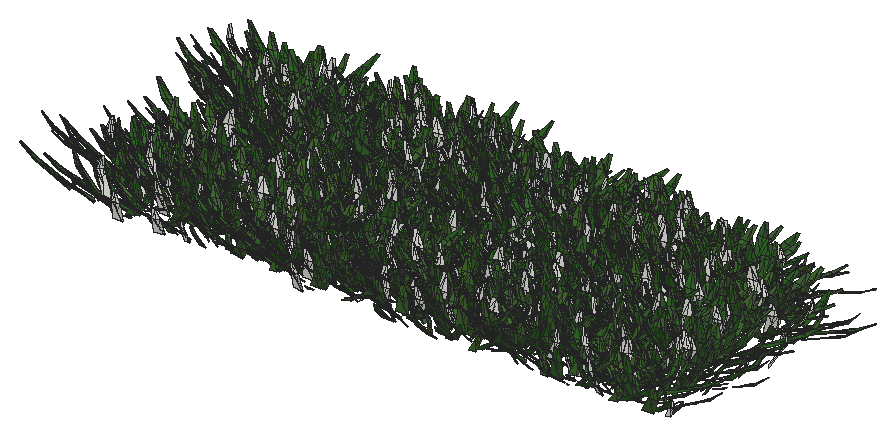
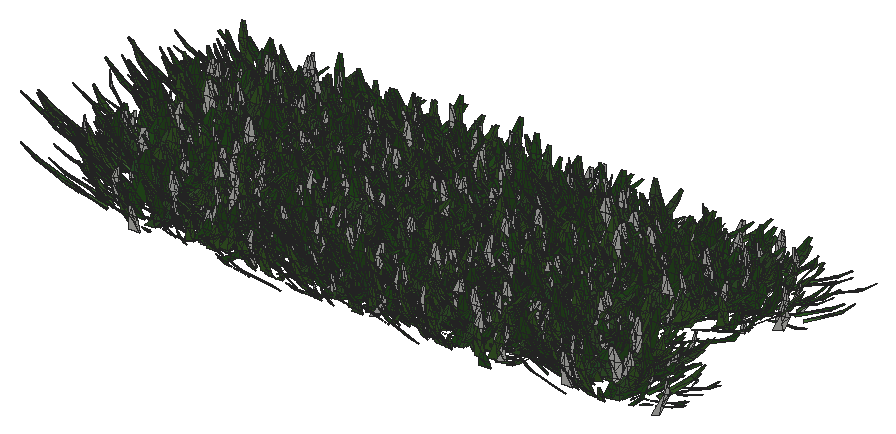
# SketchUp Ruby script. Lengths in inches.
U = 1.inch
M = Sketchup.active_model
def pt(a) = Geom::Point3d.new(a.map { |v| v * U })
def face(e, loops, mat)
  f = e.add_face(loops[0].map { |a| pt(a) })
  loops[1..].each { |l| e.add_face(l.map { |a| pt(a) }).erase! }
  f.material = f.back_material = mat if mat
  f
end
# faces: each face lists its corners as indices into pts; further lists are holes
def faces(e, pts, list, mat = nil) = list.each { |f| face(e, (f[0].is_a?(Array) ? f : [f]).map { |l| l.map { |i| pts[i] } }, mat) }
# xy, xz, yz: faces in a plane at the given z, y or x. An outline is a flat list of corners, or four numbers for a rectangle; further outlines are holes
def ring(l) = l.size == 4 ? [[l[0], l[1]], [l[2], l[1]], [l[2], l[3]], [l[0], l[3]]] : l.each_slice(2).to_a
def flat(e, list, mat, &to3) = list.each { |f| face(e, (f[0].is_a?(Array) ? f : [f]).map { |l| ring(l).map { |u, v| to3.(u, v) } }, mat) }
def xy(e, z, list, mat = nil) = flat(e, list, mat) { |x, y| [x, y, z] }
def xz(e, y, list, mat = nil) = flat(e, list, mat) { |x, z| [x, y, z] }
def yz(e, x, list, mat = nil) = flat(e, list, mat) { |y, z| [x, y, z] }
def lines(e, pts, list) = list.each { |a, b| e.add_line(pt(pts[a]), pt(pts[b])) }
# prism: a flat outline (further loops are holes) pulled along v
def prism(e, loops, v, mat = nil)
  f = face(e, loops, mat); d = Geom::Vector3d.new(v.map { |x| x * U })
  f.pushpull(f.normal.samedirection?(d) ? d.length : -d.length)
end
def box(e, o, s, mat = nil) = prism(e, [[o, [o[0] + s[0], o[1], o[2]], [o[0] + s[0], o[1] + s[1], o[2]], [o[0], o[1] + s[1], o[2]]]], [0, 0, s[2]], mat)
def at(x, y, z, deg = 0) = Geom::Transformation.translation(pt([x, y, z])) * Geom::Transformation.rotation(ORIGIN, Z_AXIS, deg.degrees)
def axes(o, x, y, z) = Geom::Transformation.new([*x, 0, *y, 0, *z, 0, *pt(o).to_a, 1])
def part(name) = M.definitions.add(name)
# library, detail: a bought-in or finely detailed component or shape, given as its bounding box
def library(name, o, s) = part(name).tap { |d| box(d.entities, o, s) }
def detail(e, o, s) = box(e.add_group.entities, o, s)
def put(e, d, t, mat = nil) = e.add_instance(d, t).tap { |i| i.material = mat if mat }
def group(e, t, mat = nil) = e.add_group.tap { |g| g.transformation = t; g.material = mat if mat }.entities
root = M.entities
M.materials.add("Material82").color = [68, 110, 58]
M.materials.add("Material83").color = [48, 90, 38]
M.materials.add("Material84").color = [68, 110, 48]
M.materials.add("Material85").color = [48, 90, 48]
M.materials.add("Material86").color = [58, 110, 58]
M.materials.add("Material87").color = [58, 90, 38]
M.materials.add("Material88").color = [68, 100, 58]
M.materials.add("Material89").color = [48, 100, 38]
c1 = part("grass00")
p = [[-0.6875,0.15,0],[-0.56,0.08,5.52],[-0.04,0.03,2.76],[0.48,-0.02,0],[0.35,-0.02,5.52],[-0.1,-0.14,5.52],
  [-0.12,0.65,8.37],[-0.42,0.65,8.37]]
faces(c1.entities,p,[[0,1,2,3],[3,2,4],[1,5,2],[5,4,2],[1,6,5],[4,5,6],[7,6,1]])
c2 = part("Group16\#1")
put(c2.entities,c1,axes([1.44,-0.61,-0.01],[0.05352,0.12609,0],[-0.10704,0.04543,0.07239],[0.06664,-0.02828,0.11628]),"Material85")
put(c2.entities,c1,axes([0.76,-0.15,-0.01],[0.04676,0.24062,0],[-0.23162,0.04501,0.06642],[0.0652,-0.01267,0.23595]),"Material82")
put(c2.entities,c1,axes([0.79,0.01,-0.01],[-0.00606,0.34651,0],[-0.34381,-0.00602,0.0432],[0.04319,0.00076,0.34386]))
put(c2.entities,c1,axes([1,0.23,-0.01],[-0.07192,0.31144,0],[-0.28722,-0.06632,0.1236],[0.12043,0.02781,0.29478]),"Material84")
put(c2.entities,c1,axes([1.66,0.77,-0.01],[-0.13828,0.29651,0],[-0.21551,-0.1005,0.22471],[0.20365,0.09498,0.23779]),"Material89")
put(c2.entities,c1,axes([0.6875,0.52,-0.01],[-0.18126,0.24051,0],[-0.22746,-0.17142,0.09788],[0.07817,0.05891,0.28481]),"Material84")
put(c2.entities,c1,axes([0.68,0.78,-0.01],[-0.215,0.18688,0],[-0.12385,-0.14248,0.21334],[0.13995,0.16101,0.18878]),"Material82")
put(c2.entities,c1,axes([0.56,1,-0.01],[-0.13756,0.07624,0],[-0.06159,-0.11112,0.0927],[0.04494,0.08108,0.12705]),"Material84")
put(c2.entities,c1,axes([0.2,0.64,-0.01],[-0.23729,0.07254,0],[-0.05711,-0.18681,0.153],[0.04473,0.14632,0.19535]),"Material89")
put(c2.entities,c1,axes([0.0625,0.72,-0.01],[-0.28874,0.02525,0],[-0.02179,-0.24916,0.14647],[0.01276,0.14591,0.25012]),"Material82")
put(c2.entities,c1,axes([-0.08,0.62,-0.01],[-0.34089,-0.04187,0],[0.03255,-0.26504,0.216],[-0.02633,0.21439,0.26703]),"Material89")
put(c2.entities,c1,axes([-0.34,0.98,-0.01],[-0.14314,-0.0493,0],[0.04397,-0.12769,0.06843],[-0.02228,0.0647,0.13505]),"Material89")
put(c2.entities,c1,axes([-0.87,1.45,-0.01],[-0.23488,-0.14114,0],[0.13761,-0.22901,0.06087],[-0.03135,0.05217,0.26717]))
put(c2.entities,c1,axes([-0.72,0.77,-0.01],[-0.14208,-0.13251,0],[0.07209,-0.0773,0.16301],[-0.11118,0.11922,0.1057]),"Material89")
put(c2.entities,c1,axes([-0.62,0.43,-0.01],[-0.14845,-0.21203,0],[0.18654,-0.13061,0.12304],[-0.10079,0.07057,0.22772]),"Material82")
put(c2.entities,c1,axes([-0.68,0.29,-0.01],[-0.13639,-0.32136,0],[0.31723,-0.13464,0.05579],[-0.05136,0.0218,0.34462]),"Material83")
put(c2.entities,c1,axes([-0.64,0.125,-0.01],[-0.0458,-0.23569,0],[0.22124,-0.043,0.08276],[-0.08124,0.01579,0.22538]),"Material86")
put(c2.entities,c1,axes([-1.6,-0.03,-0.01],[0.00576,-0.32897,0],[0.27526,0.00482,0.18018],[-0.18015,-0.00315,0.2753]),"Material84")
put(c2.entities,c1,axes([-1.36,-0.31,-0.01],[0.05718,-0.24765,0],[0.18172,0.04196,0.17267],[-0.16825,-0.03885,0.1865]),"Material89")
put(c2.entities,c1,axes([-1.54,-0.72,-0.01],[0.06537,-0.14017,0],[0.13555,0.06321,0.03939],[-0.0357,-0.01665,0.14956]))
put(c2.entities,c1,axes([-1.19,-0.9,-0.01],[0.09597,-0.12735,0],[0.11214,0.08451,0.07557],[-0.06035,-0.04548,0.14042]),"Material88")
put(c2.entities,c1,axes([-0.47,-0.54,-0.01],[0.11588,-0.10072,0],[0.0618,0.0711,0.12124],[-0.07953,-0.0915,0.0942]))
put(c2.entities,c1,axes([-0.47,-0.84,-0.01],[0.11927,-0.0661,0],[0.06603,0.11913,0.00646],[-0.00313,-0.00565,0.13621]),"Material84")
put(c2.entities,c1,axes([-0.38,-1.24,-0.01],[0.28037,-0.08571,0],[0.0618,0.20215,0.20315],[-0.05939,-0.19428,0.21139]),"Material88")
put(c2.entities,c1,axes([-0.06,-0.66,-0.01],[0.22719,-0.01987,0],[0.01247,0.14255,0.17758],[-0.01547,-0.17691,0.1431]),"Material87")
put(c2.entities,c1,axes([0.11,-0.89,-0.01],[0.14882,0.01828,0],[-0.01058,0.08611,0.12229],[0.01491,-0.12138,0.08676]),"Material85")
put(c2.entities,c1,axes([0.25,-0.72,-0.01],[0.20481,0.07053,0],[-0.06206,0.18022,0.10291],[0.03351,-0.0973,0.1906]),"Material85")
put(c2.entities,c1,axes([0.85,-1.42,-0.01],[0.16481,0.09904,0],[-0.09472,0.15762,0.05616],[0.02893,-0.04814,0.18389]),"Material84")
put(c2.entities,c1,axes([1.01,-1.09,-0.01],[0.21858,0.20385,0],[-0.17495,0.1876,0.15339],[0.10462,-0.11218,0.25652]),"Material89")
put(c2.entities,c1,axes([1.01,-0.71,-0.01],[0.08733,0.12473,0],[-0.06445,0.04512,0.13037],[0.1068,-0.07477,0.07867]),"Material85")
c3 = part("Group15\#1")
put(c3.entities,c2,at(0,0,0))
c4 = part("3darcstudiotree_grass00\#1")
put(c4.entities,c3,at(0,0,0))
put(root,c4,axes([817.78,997.54,-29.74],[3.63959,0.40285,0],[-0.8944,1.25675,-0.00495],[-0.00749,0.01053,1.38942]))
put(root,c4,axes([779.66,997.18,-29.74],[-3.14741,0.41412,0],[-1.12782,-1.33315,-0.01591],[-0.02767,-0.03271,1.46774]))
put(root,c4,axes([802.03,997.39,-29.74],[-3.08585,0.75112,0],[-1.75968,-1.12437,-0.03387],[-0.09597,-0.06132,1.3548]))
put(root,c4,axes([794.67,998.27,-29.74],[3.37216,0.16863,0],[-0.47809,1.48691,-0.01144],[-0.0086,0.02673,1.7012]))
put(root,c4,axes([833.25,998.54,-29.74],[4.62364,0.41674,0],[-0.83657,1.44354,-0.00333],[-0.00361,0.00623,1.36941]))
put(root,c4,axes([791.67,998.41,-29.74],[3.38325,1.26435,0],[-2.73925,1.14001,-0.00751],[-0.0314,0.01307,1.8142]))
put(root,c4,axes([783.74,998.28,-29.74],[-3.54635,0.32604,0],[-1.06041,-1.79388,-0.06463],[-0.05576,-0.09432,1.33032]))
put(root,c4,axes([811.51,998.95,-29.74],[-1.14276,-1.73672,0],[3.49011,-0.35717,-0.03225],[0.18285,-0.01871,1.58326]))
put(root,c4,axes([829.91,999.05,-29.74],[3.63873,-0.8009,0],[1.86273,1.31624,-0.03495],[0.11311,0.07993,1.90256]))
put(root,c4,axes([839.23,999.17,-29.74],[-1.8058,1.22943,0],[-3.0103,-0.68768,-0.02138],[-0.11593,-0.02648,1.63406]))
put(root,c4,axes([817.96,999.67,-29.74],[-1.39646,-1.43145,0],[3.7454,-0.56828,-0.0371],[0.22587,-0.03427,1.96201]))
put(root,c4,axes([805.49,999.49,-29.74],[-3.39608,-0.38473,0],[1.21289,-1.66516,-0.05258],[0.08123,-0.11153,1.84274]))
put(root,c4,axes([823.47,999.74,-29.74],[-2.82588,-0.78458,0],[2.18733,-1.22531,-0.03828],[0.15336,-0.08591,1.98208]))
put(root,c4,axes([799.14,999.59,-29.74],[-4.11359,0.33172,0],[-0.73599,-1.4195,-0.0347],[-0.04072,-0.07853,1.61275]))
put(root,c4,axes([799.8125,1000.4,-29.74],[2.00643,-1.16557,0],[2.7626,0.73963,-0.03969],[0.18592,0.04978,1.41714]))
put(root,c4,axes([797.0625,1000.67,-29.74],[-0.92987,-1.7368,0],[3.78348,-0.31505,-0.00703],[0.03581,-0.00298,1.50812]))
put(root,c4,axes([833.46,1000.76,-29.74],[2.37064,0.94684,0],[-3.28047,1.27743,-0.04002],[-0.15051,0.05861,1.82631]))
put(root,c4,axes([822.39,1001.11,-29.74],[-0.85576,-1.5606,0],[4.52661,-0.38605,-0.05631],[0.21879,-0.01866,1.37991]))
put(root,c4,axes([783.08,1000.78,-29.74],[-3.5543,0.89209,0],[-1.79933,-1.11498,-0.04609],[-0.16829,-0.10428,1.7083]))
put(root,c4,axes([812.29,1000.94,-29.74],[-4.19905,0.34301,0],[-0.96105,-1.82979,-0.05761],[-0.05651,-0.10759,1.71741]))
put(root,c4,axes([817.2,1001.26,-29.74],[1.4538,1.50227,0],[-4.10712,0.61817,-0.00597],[-0.03083,0.00464,1.82255]))
put(root,c4,axes([807.09,1001.8,-29.74],[3.76801,-0.42175,0],[1.14915,1.59678,-0.03157],[0.04846,0.06733,1.77323]))
put(root,c4,axes([827.78,1001.65,-29.74],[-2.807,-0.90771,0],[2.30635,-1.10925,-0.04795],[0.15506,-0.07458,1.39039]))
put(root,c4,axes([778.45,1001.8125,-29.74],[3.03313,0.50579,0],[-1.37798,1.28522,-0.04149],[-0.11611,0.10829,1.90578]))
put(root,c4,axes([788.75,1001.6875,-29.74],[0.41174,1.83159,0],[-3.96576,0.13865,-0.0152],[-0.08151,0.00285,1.60635]))
put(root,c4,axes([778.38,1002.9375,-29.74],[4.0409,0.57443,0],[-1.45336,1.59011,-0.05978],[-0.09434,0.10321,1.49495]))
put(root,c4,axes([818.54,1003.17,-29.74],[3.28196,0.81984,0],[-2.45781,1.53025,-0.01012],[-0.02495,0.01554,1.58691]))
put(root,c4,axes([782.26,1002.9,-29.74],[-4.1133,-0.05921,0],[0.15009,-1.6218,-0.04384],[0.00865,-0.09349,1.66887]))
put(root,c4,axes([838.32,1003.15,-29.74],[1.90217,1.207,0],[-3.00756,0.73717,-0.00184],[-0.00944,0.00231,1.60144]))
put(root,c4,axes([801.09,1003.25,-29.74],[3.28108,0.9921,0],[-2.06723,1.06332,-0.03117],[-0.09708,0.04994,1.30357]))
put(root,c4,axes([789.97,1003.66,-29.74],[1.64327,-1.14246,0],[4.09949,0.91708,-0.03953],[0.17253,0.0386,1.77239]))
put(root,c4,axes([835.82,1003.49,-29.74],[2.92133,1.34194,0],[-2.9494,0.99861,-0.03135],[-0.14252,0.04825,1.74596]))
put(root,c4,axes([794.43,1003.95,-29.74],[1.00632,-1.60929,0],[3.83281,0.37276,-0.00763],[0.0458,0.00445,1.82848]))
put(root,c4,axes([806.04,1004.0625,-29.74],[3.61578,-1.02121,0],[2.66994,1.47029,-0.04389],[0.14306,0.07878,1.92393]))
put(root,c4,axes([827.79,1003.79,-29.74],[2.97603,0.7742,0],[-2.07464,1.24033,-0.03997],[-0.14341,0.08574,1.84008]))
put(root,c4,axes([812.93,1004.14,-29.74],[0.12061,-1.58998,0],[4.18389,0.04936,-0.01737],[0.08566,0.00101,1.54781]))
put(root,c4,axes([824.48,1004.12,-29.74],[-1.60743,-1.14355,0],[3.95374,-0.86436,-0.00731],[0.03731,-0.00816,1.97847]))
put(root,c4,axes([826.84,1004.83,-29.74],[3.2807,-0.61041,0],[1.81668,1.51857,-0.02435],[0.05518,0.04613,1.69455]))
put(root,c4,axes([837.62,1005.08,-29.74],[3.15887,-0.80876,0],[1.92191,1.16751,-0.02789],[0.09845,0.05981,1.71527]))
put(root,c4,axes([806.18,1005.05,-29.74],[-0.00326,-1.3732,0],[3.39922,-0.00125,-0.0371],[0.2688,-0.0001,1.84609]))
put(root,c4,axes([822.41,1004.89,-29.74],[-3.59941,0.74413,0],[-1.52837,-1.14979,-0.02232],[-0.06679,-0.05025,1.59039]))
put(root,c4,axes([789.77,1005.21,-29.74],[0.9145,1.75116,0],[-3.69114,0.2998,-0.03105],[-0.20233,0.01643,1.87912]))
put(root,c4,axes([783.78,1005.54,-29.74],[-2.34222,-1.01748,0],[3.28821,-1.17726,-0.05879],[0.21723,-0.07777,1.66118]))
put(root,c4,axes([779.43,1005.81,-29.74],[1.55138,-1.30688,0],[2.99369,0.55272,-0.04141],[0.29892,0.05519,1.97468]))
put(root,c4,axes([818.47,1005.58,-29.74],[-1.85188,1.07885,0],[-3.29338,-0.87924,-0.00267],[-0.01201,-0.00321,1.62102]))
put(root,c4,axes([794.96,1006.01,-29.74],[3.42011,0.99957,0],[-2.24279,1.19352,-0.03152],[-0.09807,0.05219,1.47514]))
put(root,c4,axes([834.9,1005.85,-29.74],[-3.64839,-0.0594,0],[0.18827,-1.79867,-0.05407],[0.01098,-0.10487,1.68402]))
put(root,c4,axes([798.8,1006.3,-29.74],[0.26665,1.72733,0],[-3.78087,0.09078,-0.02381],[-0.14887,0.00357,1.77807]))
put(root,c4,axes([812.48,1006.3,-29.74],[-0.34365,1.56469,0],[-3.45908,-0.11816,-0.04948],[-0.26965,-0.00921,1.42361]))
put(root,c4,axes([805.92,1006.94,-29.74],[-0.07574,-1.47303,0],[4.38332,-0.03505,-0.05384],[0.21677,-0.00173,1.32332]))
put(root,c4,axes([790.89,1007.13,-29.74],[0.23576,-1.73441,0],[4.70751,0.09952,-0.00697],[0.03732,0.00079,1.89407]))
put(root,c4,axes([838.45,1007.0625,-29.74],[-3.60106,0.31713,0],[-0.9107,-1.60836,-0.00123],[-0.0017,-0.003,1.99006]))
put(root,c4,axes([821.18,1007.84,-29.74],[-0.83235,-1.28841,0],[3.31595,-0.33318,-0.03395],[0.19708,-0.0198,1.53644]))
put(root,c4,axes([812.79,1007.83,-29.74],[4.55756,-0.02191,0],[0.04205,1.36049,-0.04731],[0.00354,0.1146,1.58849]))
put(root,c4,axes([802.54,1007.71,-29.74],[-4.36692,-0.69342,0],[1.6396,-1.60594,-0.01703],[0.03175,-0.0311,1.64249]))
put(root,c4,axes([835.49,1007.85,-29.74],[-4.39804,-0.22301,0],[0.45888,-1.40747,-0.03967],[0.03344,-0.10258,1.78282]))
put(root,c4,axes([818.02,1007.92,-29.74],[-3.9934,-0.49353,0],[1.06998,-1.34652,-0.00157],[0.00241,-0.00304,1.37913]))
put(root,c4,axes([797.26,1008.24,-29.74],[-2.16285,-1.07783,0],[3.1191,-0.97346,-0.00813],[0.02825,-0.00882,1.32168]))
put(root,c4,axes([784.73,1008.125,-29.74],[-3.56597,0.54096,0],[-1.21057,-1.24113,-0.01112],[-0.02689,-0.02757,1.70172]))
put(root,c4,axes([829.42,1008.49,-29.74],[-3.12571,-0.7496,0],[2.43282,-1.57777,-0.06276],[0.13907,-0.09019,1.49667]))
put(root,c4,axes([819.21,1009.44,-29.74],[2.80724,-1.17226,0],[3.04027,1.13235,-0.05261],[0.16943,0.06311,1.38839]))
put(root,c4,axes([823.53,1009.32,-29.74],[3.98724,0.20884,0],[-0.61603,1.82924,-0.05242],[-0.03685,0.10943,1.87281]))
put(root,c4,axes([795.02,1009.29,-29.74],[-2.49579,-0.85332,0],[2.16334,-0.98408,-0.00893],[0.04692,-0.02134,1.98619]))
put(root,c4,axes([829.03,1009.21,-29.74],[-0.65898,1.54379,0],[-3.85922,-0.25621,-0.04712],[-0.21087,-0.014,1.33133]))
put(root,c4,axes([783.19,1009.15,-29.74],[-1.96915,1.54328,0],[-4.06414,-0.80652,-0.00338],[-0.01619,-0.00321,1.82725]))
put(root,c4,axes([838.22,1010.09,-29.74],[-0.6545,-1.64207,0],[4.59681,-0.28496,-0.0381],[0.20859,-0.01293,1.93318]))
put(root,c4,axes([804.89,1010.12,-29.74],[-3.35579,-1.19548,0],[2.90415,-1.2679,-0.0585],[0.2305,-0.10063,1.90866]))
put(root,c4,axes([799.49,1009.94,-29.74],[1.02208,1.31259,0],[-4.10151,0.49672,-0.03259],[-0.17155,0.02078,1.77089]))
put(root,c4,axes([810.4375,1010.25,-29.74],[-1.37112,-1.31689,0],[3.73876,-0.60543,-0.04381],[0.2334,-0.0378,1.74465]))
put(root,c4,axes([790.03,1009.94,-29.74],[1.28043,1.73979,0],[-3.30316,0.37809,-0.03743],[-0.19576,0.02241,1.40382]))
put(root,c4,axes([831.98,1010.07,-29.74],[-1.11481,1.68554,0],[-3.85911,-0.39697,-0.04083],[-0.25467,-0.0262,1.92702]))
put(root,c4,axes([835.74,1011.3,-29.74],[4.4065,0.29877,0],[-0.73465,1.68517,-0.00744],[-0.00712,0.01634,1.83611]))
put(root,c4,axes([821.52,1011.46,-29.74],[-0.43709,-1.41781,0],[4.63894,-0.22243,-0.04217],[0.16902,-0.0081,1.41426]))
put(root,c4,axes([829.64,1011.53,-29.74],[-2.31531,-0.95478,0],[2.79879,-1.05558,-0.03327],[0.10847,-0.04091,1.30962]))
put(root,c4,axes([790.6875,1011.8125,-29.74],[-3.49986,-0.57002,0],[1.44663,-1.38143,-0.04671],[0.11633,-0.11108,1.85324]))
put(root,c4,axes([795.34,1011.56,-29.74],[-3.56783,-0.13568,0],[0.42403,-1.73414,-0.0118],[0.00459,-0.01877,1.34216]))
put(root,c4,axes([812.04,1011.86,-29.74],[1.76415,1.1719,0],[-3.51067,0.82196,-0.05173],[-0.20066,0.04698,1.38038]))
put(root,c4,axes([786.07,1012.2,-29.74],[3.28347,0.12106,0],[-0.38901,1.64106,-0.04931],[-0.02254,0.09507,1.538]))
put(root,c4,axes([805.9,1011.93,-29.74],[-3.58969,-0.07657,0],[0.18796,-1.37056,-0.00522],[0.00152,-0.01105,1.40302]))
put(root,c4,axes([800.72,1012.74,-29.74],[-2.85144,-1.16634,0],[2.50888,-0.95396,-0.03577],[0.14723,-0.05598,1.49339]))
put(root,c4,axes([818.5,1012.85,-29.74],[-3.70101,0.79314,0],[-2.22235,-1.61286,-0.04664],[-0.10432,-0.07571,1.63424]))
put(root,c4,axes([811.48,1013.69,-29.74],[-2.51613,1.14478,0],[-2.79457,-0.95529,-0.04719],[-0.16752,-0.05727,1.30223]))
put(root,c4,axes([786.05,1013.84,-29.74],[-3.8899,-0.78174,0],[2.11548,-1.63718,-0.02171],[0.04442,-0.03438,1.57387]))
put(root,c4,axes([800.4,1014.18,-29.74],[-1.26006,-1.32624,0],[4.43512,-0.65537,-0.00645],[0.02239,-0.00331,1.31612]))
put(root,c4,axes([788.87,1013.81,-29.74],[-3.55041,0.9087,0],[-2.02381,-1.22981,-0.02727],[-0.0752,-0.0457,1.41127]))
put(root,c4,axes([822.65,1014.14,-29.74],[-2.86852,-0.72551,0],[1.94813,-1.19796,-0.01822],[0.05809,-0.03572,1.59761]))
put(root,c4,axes([793.39,1014.48,-29.74],[-0.24051,-1.38856,0],[3.98568,-0.10737,-0.04502],[0.19517,-0.00526,1.30109]))
put(root,c4,axes([828.62,1014.52,-29.74],[1.80555,1.12349,0],[-3.92794,0.98179,-0.01772],[-0.05919,0.0148,1.37883]))
put(root,c4,axes([816.82,1014.75,-29.74],[3.1901,1.34772,0],[-3.0794,1.13365,-0.04297],[-0.19725,0.07262,1.98261]))
put(root,c4,axes([806.74,1014.93,-29.74],[-3.3619,-0.88005,0],[2.60897,-1.55009,-0.03911],[0.08798,-0.05227,1.43856]))
put(root,c4,axes([835.79,1014.74,-29.74],[-3.86294,0.12208,0],[-0.37038,-1.82279,-0.02116],[-0.00872,-0.04291,1.79229]))
put(root,c4,axes([794.68,1016.09,-29.74],[4.22834,-0.67564,0],[1.61938,1.57623,-0.01357],[0.03127,0.03043,1.98263]))
put(root,c4,axes([800.05,1015.97,-29.74],[0.22416,-1.4452,0],[4.13727,0.09981,-0.05271],[0.23324,0.00563,1.37729]))
put(root,c4,axes([813.49,1016,-29.74],[-3.70247,-0.49757,0],[1.50858,-1.74588,-0.06303],[0.09341,-0.1081,1.61067]))
put(root,c4,axes([784.0625,1016.24,-29.74],[4.24476,0.21314,0],[-0.43337,1.34235,-0.04636],[-0.04216,0.1306,1.85211]))
put(root,c4,axes([791.78,1016.7,-29.74],[4.08655,-0.74198,0],[1.4526,1.2443,-0.00355],[0.00912,0.00781,1.60125]))
put(root,c4,axes([829.71,1016.23,-29.74],[-3.94904,-0.28889,0],[0.74698,-1.58808,-0.00704],[0.00779,-0.01657,1.86241]))
put(root,c4,axes([835.85,1016.95,-29.74],[4.62049,-0.36242,0],[0.91883,1.82189,-0.02703],[0.02558,0.05072,1.71263]))
put(root,c4,axes([820.95,1017.05,-29.74],[3.88367,-0.39615,0],[1.13822,1.73547,-0.04841],[0.06323,0.0964,1.77682]))
put(root,c4,axes([817.55,1016.47,-29.74],[-1.78787,1.37846,0],[-3.47115,-0.7002,-0.05082],[-0.20934,-0.04223,1.35221]))
put(root,c4,axes([839.23,1016.97,-29.74],[-1.11998,1.52641,0],[-4.36702,-0.49835,-0.06381],[-0.30025,-0.03426,1.66913]))
put(root,c4,axes([779.79,1017.29,-29.74],[-0.77153,1.33479,0],[-3.28421,-0.29525,-0.03421],[-0.24787,-0.02228,1.87625]))
put(root,c4,axes([804.31,1017.26,-29.74],[-1.26035,1.30994,0],[-3.37363,-0.50484,-0.03389],[-0.19382,-0.029,1.65454]))
put(root,c4,axes([795.66,1017.86,-29.74],[3.74003,-0.3626,0],[0.86697,1.39078,-0.02888],[0.04393,0.07047,1.73467]))
put(root,c4,axes([810.24,1018.03,-29.74],[3.65327,1.04493,0],[-2.10749,1.14596,-0.01189],[-0.03901,0.02121,1.50367]))
put(root,c4,axes([835.54,1018.36,-29.74],[-2.13062,-1.66467,0],[3.82642,-0.7617,-0.02075],[0.09652,-0.01921,1.67433]))
put(root,c4,axes([783.99,1018.52,-29.74],[-0.28709,-1.61704,0],[4.14071,-0.11434,-0.04142],[0.22933,-0.00633,1.72685]))
put(root,c4,axes([830.44,1018.02,-29.74],[-2.45667,1.24552,0],[-3.48685,-1.06965,-0.01031],[-0.04097,-0.01257,1.66779]))
put(root,c4,axes([837.59,1018.34,-29.74],[-4.37191,-0.09188,0],[0.22077,-1.63377,-0.04256],[0.01218,-0.09013,1.67228]))
put(root,c4,axes([779.27,1019.15,-29.74],[4.14328,-0.46419,0],[1.00154,1.39037,-0.02465],[0.03463,0.04808,1.41248]))
put(root,c4,axes([788.42,1018.78,-29.74],[1.12356,1.5327,0],[-3.46853,0.39546,-0.04889],[-0.25471,0.02904,1.46761]))
put(root,c4,axes([821.04,1019.04,-29.74],[1.48622,1.27925,0],[-3.96463,0.71638,-0.00338],[-0.01448,0.00262,1.53978]))
put(root,c4,axes([801.4,1019.39,-29.74],[-0.17296,-1.31916,0],[4.52056,-0.09218,-0.00424],[0.01978,-0.0004,1.58408]))
put(root,c4,axes([816.82,1019.15,-29.74],[-3.91187,0.00169,0],[-0.00401,-1.44027,-0.04481],[-0.00031,-0.10997,1.70362]))
put(root,c4,axes([804.57,1019.34,-29.74],[-3.17197,-0.90891,0],[2.49685,-1.35522,-0.03763],[0.13517,-0.07337,1.94544]))
put(root,c4,axes([828.02,1020.04,-29.74],[-1.43959,-1.62411,0],[3.7168,-0.5124,-0.03865],[0.23963,-0.03303,1.9383]))
put(root,c4,axes([818.3,1020.17,-29.74],[-3.49916,1.06741,0],[-2.60054,-1.32589,-0.05181],[-0.14447,-0.07366,1.45196]))
put(root,c4,axes([783.54,1020.69,-29.74],[3.55843,0.77732,0],[-2.07504,1.47739,-0.02111],[-0.0608,0.04329,1.90804]))
put(root,c4,axes([790.53,1020.63,-29.74],[2.41483,0.92576,0],[-3.06998,1.24547,-0.04673],[-0.14351,0.05822,1.45453]))
put(root,c4,axes([807.39,1020.61,-29.74],[2.09185,1.03032,0],[-2.8732,0.90727,-0.01526],[-0.08429,0.02662,1.9517]))
put(root,c4,axes([811.48,1021.46,-29.74],[3.21656,-1.06764,0],[2.25071,1.05463,-0.04982],[0.17505,0.08203,1.4295]))
put(root,c4,axes([834.41,1020.76,-29.74],[-3.05865,1.0781,0],[-2.78611,-1.22937,-0.02716],[-0.07662,-0.03381,1.32671]))
put(root,c4,axes([780.14,1020.83,-29.74],[-1.91367,1.54924,0],[-4.25661,-0.81775,-0.00711],[-0.02422,-0.00465,1.34501]))
put(root,c4,axes([824.5,1021.04,-29.74],[-3.32772,0.28661,0],[-0.75668,-1.36642,-0.01018],[-0.01111,-0.02006,1.35975]))
put(root,c4,axes([798.77,1021.3,-29.74],[-2.99545,-1.01525,0],[2.44315,-1.12112,-0.00129],[0.00439,-0.00201,1.46122]))
put(root,c4,axes([796.68,1021.61,-29.74],[-2.35271,1.42324,0],[-3.1761,-0.81658,-0.00573],[-0.02769,-0.00712,1.63969]))
put(root,c4,axes([790.97,1022.63,-29.74],[4.28624,-0.48224,0],[1.29741,1.79351,-0.04256],[0.05122,0.07081,1.55488]))
put(root,c4,axes([823.03,1022.83,-29.74],[1.63817,-1.67164,0],[3.7967,0.57868,-0.011],[0.05001,0.00762,1.48653]))
put(root,c4,axes([782.83,1022.85,-29.74],[3.65348,-0.50094,0],[1.24961,1.41744,-0.02118],[0.04225,0.04793,1.73224]))
put(root,c4,axes([794.97,1023.11,-29.74],[2.15184,-1.02148,0],[3.44742,1.1295,-0.00974],[0.03611,0.01183,1.619]))
put(root,c4,axes([816.93,1022.84,-29.74],[-3.74528,-0.54225,0],[1.29092,-1.38673,-0.02574],[0.04375,-0.047,1.38465]))
put(root,c4,axes([811.06,1023.26,-29.74],[-0.8424,-1.2576,0],[4.34376,-0.45254,-0.01354],[0.07406,-0.00772,1.90468]))
put(root,c4,axes([833.33,1022.86,-29.74],[-3.30618,0.81403,0],[-2.41899,-1.52802,-0.02972],[-0.07466,-0.04716,1.62371]))
put(root,c4,axes([828.72,1023.03,-29.74],[-3.81782,0.15844,0],[-0.49654,-1.86087,-0.00853],[-0.00435,-0.0163,1.7318]))
put(root,c4,axes([778.25,1023.76,-29.74],[3.09052,1.16305,0],[-2.75216,1.13741,-0.00767],[-0.03246,0.01341,1.8325]))
put(root,c4,axes([805.97,1023.61,-29.74],[-3.78052,0.58265,0],[-1.19847,-1.20943,-0.02866],[-0.07958,-0.08031,1.88291]))
put(root,c4,axes([799.49,1023.8,-29.74],[2.93363,1.22701,0],[-2.56818,0.95498,-0.02839],[-0.14721,0.05474,1.88589]))
put(root,c4,axes([832.5,1024.94,-29.74],[3.83562,-0.64652,0],[1.50566,1.38929,-0.01454],[0.02594,0.02394,1.30369]))
put(root,c4,axes([791.31,1024.48,-29.74],[0.63995,1.63517,0],[-3.50377,0.21327,-0.04631],[-0.28502,0.01735,1.65491]))
put(root,c4,axes([824.53,1024.55,-29.74],[-0.30333,1.33059,0],[-3.40704,-0.1208,-0.0349],[-0.19211,-0.00681,1.41691]))
put(root,c4,axes([816.86,1024.8,-29.74],[2.25108,1.29367,0],[-3.07657,0.83262,-0.0512],[-0.2098,0.05678,1.38975]))
put(root,c4,axes([810.53,1025.05,-29.74],[3.43468,1.02641,0],[-2.59272,1.34938,-0.0181],[-0.04577,0.02382,1.34745]))
put(root,c4,axes([806.96,1024.99,-29.74],[-2.81078,-0.75848,0],[2.18011,-1.25652,-0.01797],[0.04803,-0.02768,1.36964]))
put(root,c4,axes([795.67,1025.14,-29.74],[2.54513,1.12368,0],[-2.54126,0.89522,-0.01423],[-0.07597,0.02676,1.82816]))
